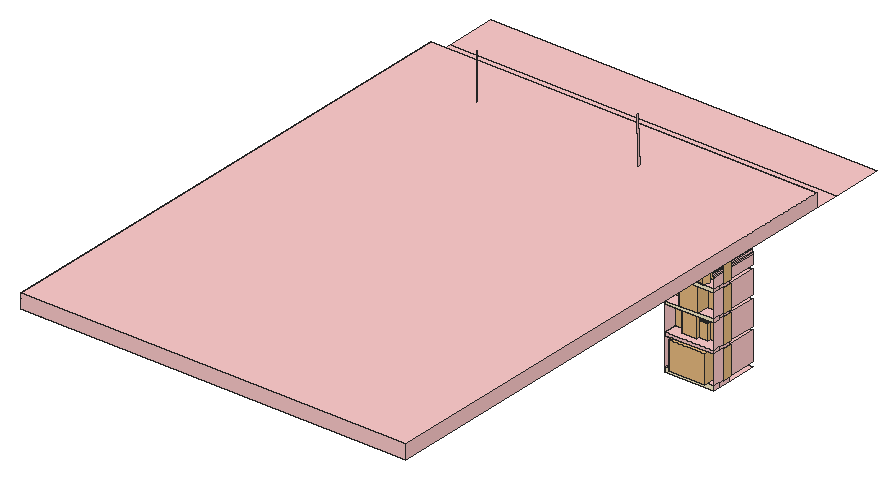
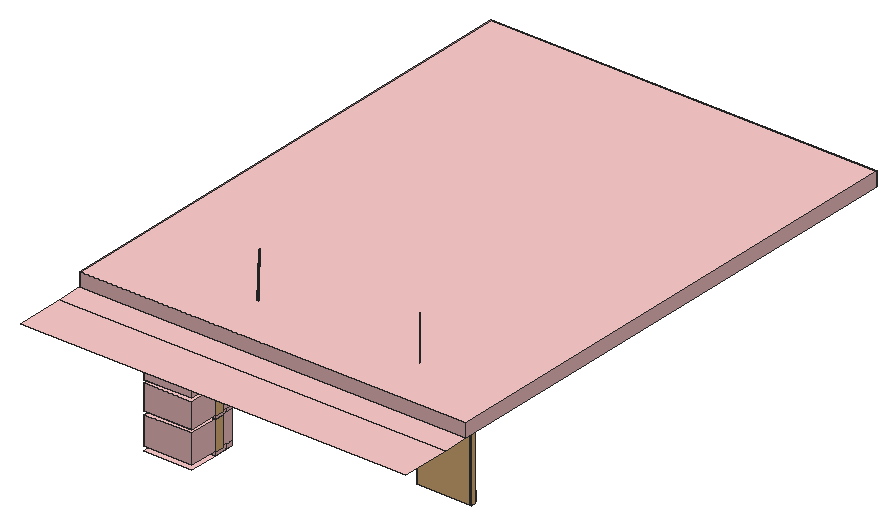
# SketchUp Ruby script. Lengths in inches.
U = 1.inch
M = Sketchup.active_model
def pt(a) = Geom::Point3d.new(a.map { |v| v * U })
def face(e, loops, mat)
  f = e.add_face(loops[0].map { |a| pt(a) })
  loops[1..].each { |l| e.add_face(l.map { |a| pt(a) }).erase! }
  f.material = f.back_material = mat if mat
  f
end
# faces: each face lists its corners as indices into pts; further lists are holes
def faces(e, pts, list, mat = nil) = list.each { |f| face(e, (f[0].is_a?(Array) ? f : [f]).map { |l| l.map { |i| pts[i] } }, mat) }
# xy, xz, yz: faces in a plane at the given z, y or x. An outline is a flat list of corners, or four numbers for a rectangle; further outlines are holes
def ring(l) = l.size == 4 ? [[l[0], l[1]], [l[2], l[1]], [l[2], l[3]], [l[0], l[3]]] : l.each_slice(2).to_a
def flat(e, list, mat, &to3) = list.each { |f| face(e, (f[0].is_a?(Array) ? f : [f]).map { |l| ring(l).map { |u, v| to3.(u, v) } }, mat) }
def xy(e, z, list, mat = nil) = flat(e, list, mat) { |x, y| [x, y, z] }
def xz(e, y, list, mat = nil) = flat(e, list, mat) { |x, z| [x, y, z] }
def yz(e, x, list, mat = nil) = flat(e, list, mat) { |y, z| [x, y, z] }
def lines(e, pts, list) = list.each { |a, b| e.add_line(pt(pts[a]), pt(pts[b])) }
# prism: a flat outline (further loops are holes) pulled along v
def prism(e, loops, v, mat = nil)
  f = face(e, loops, mat); d = Geom::Vector3d.new(v.map { |x| x * U })
  f.pushpull(f.normal.samedirection?(d) ? d.length : -d.length)
end
def box(e, o, s, mat = nil) = prism(e, [[o, [o[0] + s[0], o[1], o[2]], [o[0] + s[0], o[1] + s[1], o[2]], [o[0], o[1] + s[1], o[2]]]], [0, 0, s[2]], mat)
def at(x, y, z, deg = 0) = Geom::Transformation.translation(pt([x, y, z])) * Geom::Transformation.rotation(ORIGIN, Z_AXIS, deg.degrees)
def axes(o, x, y, z) = Geom::Transformation.new([*x, 0, *y, 0, *z, 0, *pt(o).to_a, 1])
def part(name) = M.definitions.add(name)
# library, detail: a bought-in or finely detailed component or shape, given as its bounding box
def library(name, o, s) = part(name).tap { |d| box(d.entities, o, s) }
def detail(e, o, s) = box(e.add_group.entities, o, s)
def put(e, d, t, mat = nil) = e.add_instance(d, t).tap { |i| i.material = mat if mat }
def group(e, t, mat = nil) = e.add_group.tap { |g| g.transformation = t; g.material = mat if mat }.entities
root = M.entities
M.materials.add("[Color A01]").color = [255, 204, 204]
M.materials.add("[Color D01]1").color = [255, 242, 204]
c1 = library("Group\#4",[-0.5,-0.5,0],[21.8125,3.84,12.3125])
c2 = library("ADORNOS+LIVROS+PLANTA+CELULAR+ÓCULOS",[6.19,-1.3125,-0.22],[15.35,11.9,12.07])
c3 = library("KARE 65351 Vase Hole Alu Bottle ( Vase Hole Alu Bottle )",[-6.15,-1.29,0],[12.3,2.58,18.11])
c4 = library("Group\#3",[-0.5,-0.5,0],[21.8125,3.84,10.8])
c5 = library("Group\#14",[-0.5,-0.5,0],[1,1.5625,29.57])
c6 = library("Group\#17",[-0.5,-0.5,0],[23.7,1.8125,29.57])
c7 = library("Potted plant pair",[-0.125,-0.11,0],[4.84,5.4,5.74])
c8 = library("Group\#2",[-0.5,-0.5,0],[21.8125,3.84,10.1])
c9 = library("barco decoracao",[-2.7,-0.66,0],[5.68,1.18,3.95])
c10 = library("Group\#1",[-0.5,-0.5,0],[21.8125,3.84,14.58])
c11 = library("Group\#18",[-0.5,-0.5,-0.1],[70.5,1.8125,0.2])
c12 = library("Group\#19",[-0.5,-0.5,-0.1],[13.25,1.8125,0.2])
xy(root,61.32,[[127.96,188.72,148.77,197.22],[127.96,197.22,148.77,209.91]],"[Color A01]")
xy(root,63.28,[[127.96,188.72,148.77,197.22],[127.96,197.22,148.77,209.91]],"[Color A01]")
xy(root,75.6,[[127.96,188.72,148.77,197.22],[127.96,197.22,148.77,209.91]],"[Color A01]")
xy(root,77.09,[[127.96,188.72,148.77,197.22],[127.96,197.22,148.77,209.91]],"[Color A01]")
xy(root,83.24,[[14.48,199.09,15.1,199.91]],"[Color A01]")
xy(root,87.89,[[127.96,188.72,148.77,197.22],[127.96,197.22,148.77,209.91]],"[Color A01]")
xy(root,89.17,[[127.96,188.72,148.77,197.22],[127.96,197.22,148.77,209.91]],"[Color A01]")
xy(root,90.07,[[109.2,198.91,109.21,199.66,42.02,199.91,42.01,199.16]],"[Color A01]")
xy(root,99.28,[[127.96,197.22,148.77,209.91]],"[Color A01]")
xy(root,99.28,[[127.96,188.72,148.77,197.22]],"[Color D01]1")
xy(root,100.76,[[127.96,188.72,148.77,197.22],[127.96,197.22,148.77,209.91]],"[Color A01]")
xy(root,105.9375,[[107.98,197.22,107.98,197.47,37.8,197.47,37.8,199.09,121.1,199.09,121.1,197.22,119.79,197.22,119.79,197.47,119.42,197.47,119.42,197.22,118.1,197.22,118.1,197.47,117.73,197.47,117.73,197.22,116.42,197.22,116.42,197.47,116.04,197.47,116.04,197.22,114.73,197.22,114.73,197.47,114.35,197.47,114.35,197.22,113.04,197.22,113.04,197.47,112.67,197.47,112.67,197.22,111.35,197.22,111.35,197.47,110.98,197.47,110.98,197.22,109.67,197.22,109.67,197.47,109.29,197.47,109.29,197.22]],"[Color A01]")
xy(root,106.5625,[[107.46,199.09,108.85,199.66,108.85,199.09]],"[Color A01]")
xy(root,123.9375,[[0,0,0,222.04,166.625,222.04,166.625,0,156.43,0,156.43,197.22,119.79,197.22,119.79,197.47,119.42,197.47,119.42,197.22,118.1,197.22,118.1,197.47,117.73,197.47,117.73,197.22,116.42,197.22,116.42,197.47,116.04,197.47,116.04,197.22,114.73,197.22,114.73,197.47,114.35,197.47,114.35,197.22,113.04,197.22,113.04,197.47,112.67,197.47,112.67,197.22,111.35,197.22,111.35,197.47,110.98,197.47,110.98,197.22,109.67,197.22,109.67,197.47,109.29,197.47,109.29,197.22,107.98,197.22,107.98,197.47,10.19,197.47,10.19,0],[10.19,0,10.19,197.47,107.98,197.47,107.98,197.22,109.29,197.22,109.29,197.47,109.67,197.47,109.67,197.22,110.98,197.22,110.98,197.47,111.35,197.47,111.35,197.22,112.67,197.22,112.67,197.47,113.04,197.47,113.04,197.22,114.35,197.22,114.35,197.47,114.73,197.47,114.73,197.22,116.04,197.22,116.04,197.47,116.42,197.47,116.42,197.22,117.73,197.22,117.73,197.47,118.1,197.47,118.1,197.22,119.42,197.22,119.42,197.47,119.79,197.47,119.79,197.22,121.1,197.22,121.1,188.72,156.43,188.72,156.43,0],[121.1,188.72,156.43,191.53],[121.1,191.53,156.43,197.22],[0,222.04,166.625,232.97],
  [0,232.97,166.625,254.47]],"[Color A01]")
xy(root,129.9375,[[0,0,166.625,222.04]],"[Color A01]")
xz(root,0,[[0,123.9375,166.625,129.9375]],"[Color A01]")
xz(root,188.72,[[127.96,75.6,148.77,77.09]],"[Color A01]")
xz(root,188.72,[[127.96,61.32,148.77,63.28],[127.96,87.89,148.77,89.17],[127.96,99.28,148.77,100.76]],"[Color D01]1")
xz(root,197.22,[[127.96,61.32,148.77,63.28],[127.96,63.28,148.77,75.6],[127.96,75.6,148.77,77.09],[127.96,77.09,148.77,87.89],[127.96,87.89,148.77,89.17],
  [127.96,99.28,148.77,100.76],[127.96,100.76,148.77,100.76,148.77,104.93,148.75,105.47,148.71,106.01,148.64,106.55,148.54,107.09,148.41,107.62,148.26,108.14,148.08,108.66,147.87,109.16,147.63,109.65,147.375,110.13,147.09,110.59,146.78,111.04,146.45,111.48,146.1,111.89,145.72,112.28,145.33,112.66,144.91,113.01,144.48,113.35,144.03,113.65,143.57,113.9375,143.09,114.2,142.6,114.43,142.09,114.64,141.58,114.82,141.06,114.98,140.53,115.11,139.99,115.2,139.45,115.28,138.91,115.32,138.36,115.33,137.82,115.32,137.28,115.28,136.73,115.2,136.2,115.11,135.67,114.98,135.15,114.82,134.63,114.64,134.13,114.43,133.64,114.2,133.16,113.9375,132.7,113.65,132.25,113.35,131.8125,113.01,131.4,112.66,131,112.28,130.63,111.89,130.28,111.48,129.94,111.04,129.64,110.59,129.35,110.13,129.09,109.65,128.86,109.16,128.65,108.66,128.47,108.14,128.3125,107.62,128.18,107.09,128.08,106.55,128.01,106.01,127.97,105.47,127.96,104.93]],"[Color A01]")
xz(root,197.22,[[127.96,89.17,148.77,99.28],[107.98,105.9375,109.29,123.9375],[109.67,105.9375,110.98,123.9375],[111.35,105.9375,112.67,123.9375],[113.04,105.9375,114.35,123.9375],
  [114.73,105.9375,116.04,123.9375],[116.42,105.9375,117.73,123.9375],[118.1,105.9375,119.42,123.9375],[119.79,105.9375,121.1,123.9375]],"[Color D01]1")
xz(root,197.47,[[109.29,105.9375,109.67,123.9375],[110.98,105.9375,111.35,123.9375],[112.67,105.9375,113.04,123.9375],[114.35,105.9375,114.73,123.9375],[116.04,105.9375,116.42,123.9375],
  [117.73,105.9375,118.1,123.9375],[119.42,105.9375,119.79,123.9375]],"[Color A01]")
xz(root,199.09,[[107.3,105.9375,107.46,106.5625],[107.46,105.9375,121.1,106.5625]],"[Color A01]")
xz(root,199.91,[[37.8,105.9375,107.3,106.5625]],"[Color A01]")
xz(root,209.91,[[127.96,63.28,148.77,75.6],[127.96,77.09,148.77,87.89],[127.96,89.17,148.77,99.28],[127.96,100.76,127.96,104.93,127.97,105.47,128.01,106.01,128.08,106.55,128.18,107.09,128.3125,107.62,128.47,108.14,128.65,108.66,128.86,109.16,129.09,109.65,129.35,110.13,129.64,110.59,129.94,111.04,130.28,111.48,130.63,111.89,131,112.28,131.4,112.66,131.8125,113.01,132.25,113.35,132.7,113.65,133.16,113.9375,133.64,114.2,134.13,114.43,134.63,114.64,135.15,114.82,135.67,114.98,136.2,115.11,136.73,115.2,137.28,115.28,137.82,115.32,138.36,115.33,138.91,115.32,139.45,115.28,139.99,115.2,140.53,115.11,141.06,114.98,141.58,114.82,142.09,114.64,142.6,114.43,143.09,114.2,143.57,113.9375,144.03,113.65,144.48,113.35,144.91,113.01,145.33,112.66,145.72,112.28,146.1,111.89,146.45,111.48,146.78,111.04,147.09,110.59,147.375,110.13,147.63,109.65,147.87,109.16,148.08,108.66,148.26,108.14,148.41,107.62,148.54,107.09,148.64,106.55,148.71,106.01,148.75,105.47,148.77,104.93,148.77,100.76]],"[Color A01]")
xz(root,222.04,[[0,123.9375,166.625,129.9375]],"[Color A01]")
yz(root,0,[[0,123.9375,222.04,129.9375]],"[Color A01]")
yz(root,15.1,[[199.66,83.24,199.91,83.24,199.66,112.8125]],"[Color A01]")
yz(root,37.8,[[199.09,105.9375,199.09,106.5625,199.66,149.43,199.91,106.5625,199.91,105.9375]],"[Color A01]")
yz(root,107.3,[[199.09,105.9375,199.91,105.9375,199.91,106.5625,199.66,149.43,199.09,106.5625]],"[Color A01]")
yz(root,107.98,[[197.22,105.9375,197.47,123.9375]],"[Color A01]")
yz(root,109.29,[[197.22,105.9375,197.47,123.9375]],"[Color A01]")
yz(root,109.67,[[197.22,105.9375,197.47,123.9375]],"[Color A01]")
yz(root,110.98,[[197.22,105.9375,197.47,123.9375]],"[Color A01]")
yz(root,111.35,[[197.22,105.9375,197.47,123.9375]],"[Color A01]")
yz(root,112.67,[[197.22,105.9375,197.47,123.9375]],"[Color A01]")
yz(root,113.04,[[197.22,105.9375,197.47,123.9375]],"[Color A01]")
yz(root,114.35,[[197.22,105.9375,197.47,123.9375]],"[Color A01]")
yz(root,114.73,[[197.22,105.9375,197.47,123.9375]],"[Color A01]")
yz(root,116.04,[[197.22,105.9375,197.47,123.9375]],"[Color A01]")
yz(root,116.42,[[197.22,105.9375,197.47,123.9375]],"[Color A01]")
yz(root,117.73,[[197.22,105.9375,197.47,123.9375]],"[Color A01]")
yz(root,118.1,[[197.22,105.9375,197.47,123.9375]],"[Color A01]")
yz(root,119.42,[[197.22,105.9375,197.47,123.9375]],"[Color A01]")
yz(root,119.79,[[197.22,105.9375,197.47,123.9375]],"[Color A01]")
yz(root,127.96,[[188.72,61.32,191.53,63.28],[191.53,61.32,197.22,63.28],[188.72,63.28,194.375,75.6],[197.22,63.28,209.91,75.6],[188.72,75.6,191.53,77.09],
  [191.53,75.6,197.22,77.09],[188.72,77.09,194.375,87.89],[197.22,77.09,209.91,87.89],[188.72,87.89,191.53,89.17],[191.53,87.89,197.22,89.17],
  [188.72,89.17,194.375,99.28],[197.22,89.17,209.91,99.28],[188.72,99.28,191.53,100.76],[191.53,99.28,197.22,100.76],[188.72,100.76,194.375,104.93],
  [197.22,100.76,209.91,104.93]],"[Color A01]")
yz(root,148.77,[[188.72,61.32,191.53,63.28],[191.53,61.32,197.22,63.28],[188.72,63.28,194.375,75.6],[197.22,63.28,209.91,75.6],[188.72,75.6,191.53,77.09],
  [191.53,75.6,197.22,77.09],[188.72,77.09,194.375,87.89],[197.22,77.09,209.91,87.89],[188.72,87.89,191.53,89.17],[191.53,87.89,197.22,89.17],
  [188.72,89.17,194.375,99.28],[197.22,89.17,209.91,99.28],[188.72,99.28,191.53,100.76],[191.53,99.28,197.22,100.76],[188.72,100.76,194.375,104.93],
  [197.22,100.76,209.91,104.93]],"[Color A01]")
yz(root,166.625,[[0,123.9375,222.04,129.9375]],"[Color A01]")
p = [[15.1,197.47,83.24],[15.1,199.09,83.24],[15.3,199.09,86.2],[15.3,197.47,86.2],[15.88,199.09,89.11],[15.88,197.47,89.11],
  [16.83,199.09,91.93],[16.83,197.47,91.93],[18.15,199.09,94.59],[18.15,197.47,94.59],[19.79,199.09,97.06],[19.79,197.47,97.06],
  [21.75,199.09,99.29],[21.75,197.47,99.29],[23.98,199.09,101.25],[23.98,197.47,101.25],[26.45,199.09,102.9],[26.45,197.47,102.9],
  [29.12,199.09,104.21],[29.12,197.47,104.21],[31.93,199.09,105.16],[31.93,197.47,105.16],[127.97,194.375,105.47],[127.97,188.72,105.47],
  [127.96,188.72,104.93],[127.96,194.375,104.93],[148.77,194.375,104.93],[148.77,188.72,104.93],[148.75,188.72,105.47],[148.75,194.375,105.47],
  [127.96,197.22,104.93],[127.97,197.22,105.47],[127.97,209.91,105.47],[127.96,209.91,104.93],[148.75,197.22,105.47],[148.77,197.22,104.93],
  [148.77,209.91,104.93],[148.75,209.91,105.47],[34.84,199.09,105.74],[34.84,197.47,105.74],[128.01,194.375,106.01],[128.01,188.72,106.01],
  [148.71,188.72,106.01],[148.71,194.375,106.01],[128.01,197.22,106.01],[128.01,209.91,106.01],[148.71,197.22,106.01],[148.71,209.91,106.01],
  [37.8,199.09,105.9375],[37.8,197.47,105.9375],[128.08,194.375,106.55],[128.08,188.72,106.55],[148.64,188.72,106.55],[148.64,194.375,106.55],
  [128.08,197.22,106.55],[128.08,209.91,106.55],[148.64,197.22,106.55],[148.64,209.91,106.55],[128.18,194.375,107.09],[128.18,188.72,107.09],
  [148.54,188.72,107.09],[148.54,194.375,107.09],[128.18,197.22,107.09],[128.18,209.91,107.09],[148.54,197.22,107.09],[148.54,209.91,107.09],
  [108.85,199.66,106.5625],[107.46,199.66,149.43],[107.46,198.91,149.43],[108.85,198.91,106.5625],[108.85,199.09,106.5625],[107.3,199.66,149.43],
  [107.46,199.09,106.5625],[107.3,199.09,106.5625],[107.3,199.91,106.5625],[107.46,199.91,106.5625],[128.3125,194.375,107.62],[128.3125,188.72,107.62],
  [148.41,188.72,107.62],[148.41,194.375,107.62],[128.3125,197.22,107.62],[128.3125,209.91,107.62],[148.41,197.22,107.62],[148.41,209.91,107.62],
  [128.47,194.375,108.14],[128.47,188.72,108.14],[148.26,188.72,108.14],[148.26,194.375,108.14],[128.47,197.22,108.14],[128.47,209.91,108.14],
  [148.26,197.22,108.14],[148.26,209.91,108.14],[128.65,194.375,108.66],[128.65,188.72,108.66],[148.08,188.72,108.66],[148.08,194.375,108.66],
  [128.65,197.22,108.66],[128.65,209.91,108.66],[148.08,197.22,108.66],[148.08,209.91,108.66],[128.86,194.375,109.16],[128.86,188.72,109.16],
  [147.87,188.72,109.16],[147.87,194.375,109.16],[128.86,197.22,109.16],[128.86,209.91,109.16],[147.87,197.22,109.16],[147.87,209.91,109.16],
  [129.09,194.375,109.65],[129.09,188.72,109.65],[147.63,188.72,109.65],[147.63,194.375,109.65],[129.09,197.22,109.65],[129.09,209.91,109.65],
  [147.63,197.22,109.65],[147.63,209.91,109.65],[129.35,194.375,110.13],[129.35,188.72,110.13],[147.375,188.72,110.13],[147.375,194.375,110.13],
  [129.35,197.22,110.13],[129.35,209.91,110.13],[147.375,197.22,110.13],[147.375,209.91,110.13],[129.64,194.375,110.59],[129.64,188.72,110.59],
  [147.09,188.72,110.59],[147.09,194.375,110.59],[129.64,197.22,110.59],[129.64,209.91,110.59],[147.09,197.22,110.59],[147.09,209.91,110.59],
  [129.94,194.375,111.04],[129.94,188.72,111.04],[146.78,188.72,111.04],[146.78,194.375,111.04],[129.94,197.22,111.04],[129.94,209.91,111.04],
  [146.78,197.22,111.04],[146.78,209.91,111.04],[130.28,194.375,111.48],[130.28,188.72,111.48],[146.45,188.72,111.48],[146.45,194.375,111.48],
  [130.28,197.22,111.48],[130.28,209.91,111.48],[146.45,197.22,111.48],[146.45,209.91,111.48],[130.63,194.375,111.89],[130.63,188.72,111.89],
  [146.1,188.72,111.89],[146.1,194.375,111.89],[130.63,197.22,111.89],[130.63,209.91,111.89],[146.1,197.22,111.89],[146.1,209.91,111.89],
  [131,194.375,112.28],[131,188.72,112.28],[145.72,188.72,112.28],[145.72,194.375,112.28],[131,197.22,112.28],[131,209.91,112.28],
  [145.72,197.22,112.28],[145.72,209.91,112.28],[131.4,194.375,112.66],[131.4,188.72,112.66],[145.33,188.72,112.66],[145.33,194.375,112.66],
  [131.4,197.22,112.66],[131.4,209.91,112.66],[145.33,197.22,112.66],[145.33,209.91,112.66],[131.8125,194.375,113.01],[131.8125,188.72,113.01],
  [144.91,188.72,113.01],[144.91,194.375,113.01],[131.8125,197.22,113.01],[131.8125,209.91,113.01],[144.91,197.22,113.01],[144.91,209.91,113.01],
  [132.25,194.375,113.35],[132.25,188.72,113.35],[144.48,188.72,113.35],[144.48,194.375,113.35],[132.25,197.22,113.35],[132.25,209.91,113.35],
  [144.48,197.22,113.35],[144.48,209.91,113.35],[132.7,194.375,113.65],[132.7,188.72,113.65],[144.03,188.72,113.65],[144.03,194.375,113.65],
  [132.7,197.22,113.65],[132.7,209.91,113.65],[144.03,197.22,113.65],[144.03,209.91,113.65],[133.16,194.375,113.9375],[133.16,188.72,113.9375],
  [143.57,188.72,113.9375],[143.57,194.375,113.9375],[133.16,197.22,113.9375],[133.16,209.91,113.9375],[143.57,197.22,113.9375],[143.57,209.91,113.9375],
  [133.64,194.375,114.2],[133.64,188.72,114.2],[143.09,188.72,114.2],[143.09,194.375,114.2],[133.64,197.22,114.2],[133.64,209.91,114.2],
  [143.09,197.22,114.2],[143.09,209.91,114.2],[134.13,194.375,114.43],[134.13,188.72,114.43],[142.6,188.72,114.43],[142.6,194.375,114.43],
  [134.13,197.22,114.43],[134.13,209.91,114.43],[142.6,197.22,114.43],[142.6,209.91,114.43],[134.63,194.375,114.64],[134.63,188.72,114.64],
  [142.09,188.72,114.64],[142.09,194.375,114.64],[134.63,197.22,114.64],[134.63,209.91,114.64],[142.09,197.22,114.64],[142.09,209.91,114.64],
  [135.15,194.375,114.82],[135.15,188.72,114.82],[141.58,188.72,114.82],[141.58,194.375,114.82],[135.15,197.22,114.82],[135.15,209.91,114.82],
  [141.58,197.22,114.82],[141.58,209.91,114.82],[135.67,194.375,114.98],[135.67,188.72,114.98],[141.06,188.72,114.98],[141.06,194.375,114.98],
  [135.67,197.22,114.98],[135.67,209.91,114.98],[141.06,197.22,114.98],[141.06,209.91,114.98],[136.2,194.375,115.11],[136.2,188.72,115.11],
  [140.53,188.72,115.11],[140.53,194.375,115.11],[136.2,197.22,115.11],[136.2,209.91,115.11],[140.53,197.22,115.11],[140.53,209.91,115.11],
  [136.73,194.375,115.2],[136.73,188.72,115.2],[139.99,188.72,115.2],[139.99,194.375,115.2],[136.73,197.22,115.2],[136.73,209.91,115.2],
  [139.99,197.22,115.2],[139.99,209.91,115.2],[137.28,194.375,115.28],[137.28,188.72,115.28],[139.45,188.72,115.28],[139.45,194.375,115.28],
  [137.28,197.22,115.28],[137.28,209.91,115.28],[139.45,197.22,115.28],[139.45,209.91,115.28],[137.82,194.375,115.32],[137.82,188.72,115.32],
  [138.36,194.375,115.33],[138.36,188.72,115.33],[138.91,194.375,115.32],[138.91,188.72,115.32],[137.82,197.22,115.32],[137.82,209.91,115.32],
  [138.36,197.22,115.33],[138.36,209.91,115.33],[138.91,197.22,115.32],[138.91,209.91,115.32],[37.8,199.09,106.5625],[107.8,198.59,105.9375],
  [121.1,198.59,105.9375],[107.8,198.91,105.9375],[108.85,198.91,105.9375]]
faces(root,p,[[0,1,2,3],[3,2,4,5],[5,4,6,7],[7,6,8,9],[9,8,10,11],[11,10,12,13],[13,12,14,15],[15,14,16,17],
  [17,16,18,19],[19,18,20,21],[22,23,24,25],[26,27,28,29],[30,31,32,33],[34,35,36,37],[21,20,38,39],[40,41,23,22],
  [29,28,42,43],[31,44,45,32],[46,34,37,47],[39,38,48,49],[50,51,41,40],[43,42,52,53],[44,54,55,45],[56,46,47,57],
  [58,59,51,50],[53,52,60,61],[54,62,63,55],[64,56,57,65],[66,67,68,69,70],[71,67,72,73],[66,72,67],[74,75,67,71],
  [76,77,59,58],[61,60,78,79],[62,80,81,63],[82,64,65,83],[84,85,77,76],[79,78,86,87],[80,88,89,81],[90,82,83,91],
  [92,93,85,84],[87,86,94,95],[88,96,97,89],[98,90,91,99],[100,101,93,92],[95,94,102,103],[96,104,105,97],[106,98,99,107],
  [108,109,101,100],[103,102,110,111],[104,112,113,105],[114,106,107,115],[116,117,109,108],[111,110,118,119],[112,120,121,113],[122,114,115,123],
  [124,125,117,116],[119,118,126,127],[120,128,129,121],[130,122,123,131],[132,133,125,124],[127,126,134,135],[128,136,137,129],[138,130,131,139],
  [140,141,133,132],[135,134,142,143],[136,144,145,137],[146,138,139,147],[148,149,141,140],[143,142,150,151],[144,152,153,145],[154,146,147,155],
  [156,157,149,148],[151,150,158,159],[152,160,161,153],[162,154,155,163],[164,165,157,156],[159,158,166,167],[160,168,169,161],[170,162,163,171],
  [172,173,165,164],[167,166,174,175],[168,176,177,169],[178,170,171,179],[180,181,173,172],[175,174,182,183],[176,184,185,177],[186,178,179,187],
  [188,189,181,180],[183,182,190,191],[184,192,193,185],[194,186,187,195],[196,197,189,188],[191,190,198,199],[192,200,201,193],[202,194,195,203],
  [204,205,197,196],[199,198,206,207],[200,208,209,201],[210,202,203,211],[212,213,205,204],[207,206,214,215],[208,216,217,209],[218,210,211,219],
  [220,221,213,212],[215,214,222,223],[216,224,225,217],[226,218,219,227],[228,229,221,220],[223,222,230,231],[224,232,233,225],[234,226,227,235],
  [236,237,229,228],[231,230,238,239],[232,240,241,233],[242,234,235,243],[244,245,237,236],[239,238,246,247],[240,248,249,241],[250,242,243,251],
  [252,253,245,244],[247,246,254,255],[248,256,257,249],[258,250,251,259],[260,261,253,252],[255,254,262,263],[256,264,265,257],[266,258,259,267],
  [268,269,261,260],[270,271,269,268],[272,273,271,270],[263,262,273,272],[264,274,275,265],[274,276,277,275],[276,278,279,277],[278,266,267,279]],"[Color A01]")
lines(root,p,[[280,73],[281,282],[281,283],[283,284]])
put(root,c1,at(127.96,194.375,63.28),"[Color A01]")
put(root,c2,at(124.52,188.72,63.62),"[Color A01]")
put(root,c3,axes([136.19,192.07,77.09],[-0.4958,0,0],[0,0.4958,0],[0,0,0.4958]),"[Color A01]")
put(root,c3,axes([141.17,193.05,77.09],[-0.37,0,0],[0,0.37,0],[0,0,0.37]),"[Color A01]")
put(root,c4,at(127.96,194.375,77.09),"[Color A01]")
put(root,c5,at(15.1,199.09,83.24),"[Color A01]")
put(root,c6,at(15.1,199.09,83.24),"[Color A01]")
put(root,c7,axes([133.86,188.91,89.17],[1.75,0,0],[0,1.75,0],[0,0,1.75]),"[Color A01]")
put(root,c8,at(127.96,194.375,89.17),"[Color A01]")
put(root,c9,axes([138.51,192.51,100.76],[-2.28804,0.84302,0],[0.84302,2.28804,0],[0,0,2.4384]),"[Color A01]")
put(root,c10,at(127.96,194.375,100.76),"[Color A01]")
put(root,c11,at(37.8,199.09,105.9375),"[Color A01]")
put(root,c12,at(108.85,199.09,106.5625),"[Color A01]")
